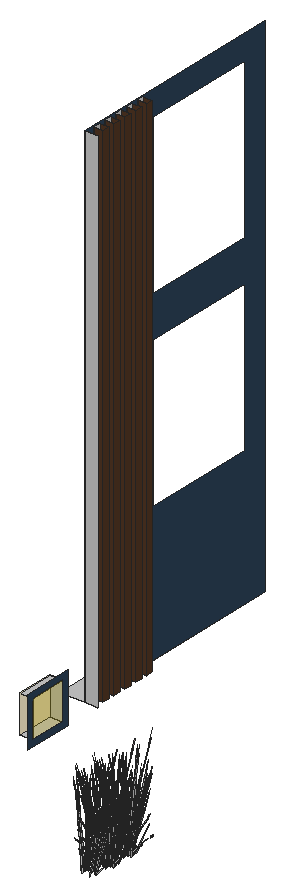
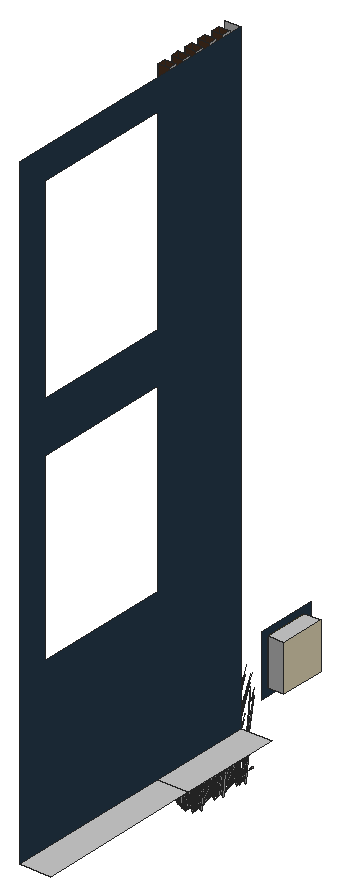
# SketchUp Ruby script. Lengths in inches.
U = 1.inch
M = Sketchup.active_model
def pt(a) = Geom::Point3d.new(a.map { |v| v * U })
def face(e, loops, mat)
  f = e.add_face(loops[0].map { |a| pt(a) })
  loops[1..].each { |l| e.add_face(l.map { |a| pt(a) }).erase! }
  f.material = f.back_material = mat if mat
  f
end
# faces: each face lists its corners as indices into pts; further lists are holes
def faces(e, pts, list, mat = nil) = list.each { |f| face(e, (f[0].is_a?(Array) ? f : [f]).map { |l| l.map { |i| pts[i] } }, mat) }
# xy, xz, yz: faces in a plane at the given z, y or x. An outline is a flat list of corners, or four numbers for a rectangle; further outlines are holes
def ring(l) = l.size == 4 ? [[l[0], l[1]], [l[2], l[1]], [l[2], l[3]], [l[0], l[3]]] : l.each_slice(2).to_a
def flat(e, list, mat, &to3) = list.each { |f| face(e, (f[0].is_a?(Array) ? f : [f]).map { |l| ring(l).map { |u, v| to3.(u, v) } }, mat) }
def xy(e, z, list, mat = nil) = flat(e, list, mat) { |x, y| [x, y, z] }
def xz(e, y, list, mat = nil) = flat(e, list, mat) { |x, z| [x, y, z] }
def yz(e, x, list, mat = nil) = flat(e, list, mat) { |y, z| [x, y, z] }
def lines(e, pts, list) = list.each { |a, b| e.add_line(pt(pts[a]), pt(pts[b])) }
# prism: a flat outline (further loops are holes) pulled along v
def prism(e, loops, v, mat = nil)
  f = face(e, loops, mat); d = Geom::Vector3d.new(v.map { |x| x * U })
  f.pushpull(f.normal.samedirection?(d) ? d.length : -d.length)
end
def box(e, o, s, mat = nil) = prism(e, [[o, [o[0] + s[0], o[1], o[2]], [o[0] + s[0], o[1] + s[1], o[2]], [o[0], o[1] + s[1], o[2]]]], [0, 0, s[2]], mat)
def at(x, y, z, deg = 0) = Geom::Transformation.translation(pt([x, y, z])) * Geom::Transformation.rotation(ORIGIN, Z_AXIS, deg.degrees)
def axes(o, x, y, z) = Geom::Transformation.new([*x, 0, *y, 0, *z, 0, *pt(o).to_a, 1])
def part(name) = M.definitions.add(name)
# library, detail: a bought-in or finely detailed component or shape, given as its bounding box
def library(name, o, s) = part(name).tap { |d| box(d.entities, o, s) }
def detail(e, o, s) = box(e.add_group.entities, o, s)
def put(e, d, t, mat = nil) = e.add_instance(d, t).tap { |i| i.material = mat if mat }
def group(e, t, mat = nil) = e.add_group.tap { |g| g.transformation = t; g.material = mat if mat }.entities
root = M.entities
M.materials.add("Carpet_04_1K").color = [43, 65, 85]
M.materials.add("D01_Frost_White").color = [255, 242, 206]
M.materials.add("Glass_Basic_01").color = [255, 228, 0]
M.materials["Glass_Basic_01"].alpha = 0.25
M.materials.add("LightPink_Translucent").color = [144, 107, 117]
M.materials["LightPink_Translucent"].alpha = 0.75
M.materials.add("Wood_Veneer_15_1K").color = [81, 54, 35]
M.materials.add("[_0053_Ivory_]").color = [200, 200, 200]
c1 = part("blade")
p = [[2.15,0.21,22],[0,0.17,0],[0.09,0.45,0],[2.18,0.31,22],[2.29,0.31,22],[0.38,0.45,0],
  [2.48,0.24,33],[2.49,0.24,33],[2.48,0.22,33]]
faces(c1.entities,p,[[0,1,2,3],[4,5,2,3],[6,3,4,7],[8,0,3,6]])
c2 = part("seeds")
p = [[0.3,-0.1,1.38],[-0.01,-0.03,1.59],[-0.01,-0.03,0.03],[0.14,-0.07,-0.07],[0.29,-0.03,3],[0.15,0.01,3.11]]
faces(c2.entities,p,[[0,1,2,3],[1,0,4,5]],"LightPink_Translucent")
c3 = part("blade with seeds")
put(c3.entities,c1,at(0,0,0))
put(c3.entities,c2,axes([2.4,0.25,30.99],[1.5799,-0.05474,1.17369],[-0.12525,1.92788,0.29478],[-0.07173,-0.02425,1.56792]))
xy(root,84,[[635.1,371.15,647.1,411.95],[648.1,375.42,652.51,378.69],[648.1,381.96,652.51,385.24],[648.1,388.51,652.51,391.78],[648.1,395.05,652.51,398.33],
  [648.1,401.6,652.51,404.87],[635.1,411.95,647.1,479.15]],"[_0053_Ivory_]")
xy(root,87,[[647.1,332.15,653.51,350.15]],"[_0053_Ivory_]")
xy(root,105,[[647.1,332.15,653.51,350.15]],"[_0053_Ivory_]")
xz(root,350.15,[[647.1,87,653.51,105]],"[_0053_Ivory_]")
xz(root,371.15,[[647.1,84,653.51,330]],"[_0053_Ivory_]")
xz(root,375.42,[[648.1,84,652.51,330]],"Wood_Veneer_15_1K")
xz(root,378.69,[[648.1,84,652.51,330]],"Wood_Veneer_15_1K")
xz(root,381.96,[[648.1,84,652.51,330]],"Wood_Veneer_15_1K")
xz(root,385.24,[[648.1,84,652.51,330]],"Wood_Veneer_15_1K")
xz(root,388.51,[[648.1,84,652.51,330]],"Wood_Veneer_15_1K")
xz(root,391.78,[[648.1,84,652.51,330]],"Wood_Veneer_15_1K")
xz(root,395.05,[[648.1,84,652.51,330]],"Wood_Veneer_15_1K")
xz(root,398.33,[[648.1,84,652.51,330]],"Wood_Veneer_15_1K")
xz(root,401.6,[[648.1,84,652.51,330]],"Wood_Veneer_15_1K")
xz(root,404.87,[[648.1,84,652.51,330]],"Wood_Veneer_15_1K")
yz(root,647.1,[[[371.15,84,479.15,330],[411.95,241.75,467.15,318],[411.95,150,467.15,222]]],"Carpet_04_1K")
yz(root,647.1,[[332.15,87,350.15,105]],"D01_Frost_White")
yz(root,648.1,[[375.42,84,378.69,330],[381.96,84,385.24,330],[388.51,84,391.78,330],[395.05,84,398.33,330],[401.6,84,404.87,330]],"[_0053_Ivory_]")
yz(root,652.51,[[375.42,84,378.69,330],[381.96,84,385.24,330],[388.51,84,391.78,330],[395.05,84,398.33,330],[401.6,84,404.87,330]],"Wood_Veneer_15_1K")
yz(root,653.51,[[[329.15,84,353.15,108],[332.15,87,350.15,105]]],"Carpet_04_1K")
yz(root,653.51,[[332.15,87,350.15,105]],"Glass_Basic_01")
put(root,c3,axes([677.18,332.05,38.6875],[0.30559,0.56943,-0.1216],[-0.54237,0.27983,-0.67495],[-0.22856,0.07513,1.02557]),"[_0053_Ivory_]")
put(root,c3,axes([681.79,334.5,38.6875],[0.03252,-0.63953,-0.1216],[0.61574,0.01748,-0.67495],[0.23714,0.04442,1.02557]),"[_0053_Ivory_]")
put(root,c3,axes([681.69,334.25,38.7],[-0.34557,-0.39372,0.35414],[0.39459,-0.37271,-0.4572],[0.20048,0.05671,0.87481]),"[_0053_Ivory_]")
put(root,c3,axes([682.32,334.12,38.37],[0.13029,-0.01064,1.74944],[0.35737,-0.48855,-0.27667],[0.23175,0.06449,0.14031]),"[_0053_Ivory_]")
put(root,c3,axes([677.11,333.64,38.39],[-0.15063,-0.57876,0.48003],[0.59087,-0.10045,0.3958],[-0.17414,0.13612,0.9933]),"[_0053_Ivory_]")
put(root,c3,axes([677,333.53,38.38],[-0.41695,-0.26447,0.0643],[0.24275,-0.37662,0.50621],[-0.13368,0.12176,0.77189]),"[_0053_Ivory_]")
put(root,c3,axes([679.55,339.63,38.37],[-0.0929,-0.08817,1.74944],[-0.61994,0.0559,-0.27667],[-0.09894,-0.21089,0.14031]),"[_0053_Ivory_]")
put(root,c3,axes([677.48,333.45,38.7],[0.52868,-0.08987,0.35414],[0.1396,0.51376,-0.4572],[-0.1515,0.13799,0.87481]),"[_0053_Ivory_]")
put(root,c3,axes([675.4375,333.22,38.36],[0.07751,0.01687,1.77383],[0.23978,0.55562,-0.16761],[-0.15867,0.14583,0.31391]),"[_0053_Ivory_]")
put(root,c3,axes([682.01,334.61,38.38],[-0.03058,0.47819,0.0643],[-0.4618,-0.01311,0.50621],[0.1769,0.05004,0.77189]),"[_0053_Ivory_]")
put(root,c3,axes([682.05,334.46,38.39],[-0.44783,0.41436,0.48003],[-0.38623,-0.44004,0.3958],[0.21011,0.07643,0.9933]),"[_0053_Ivory_]")
put(root,c3,axes([682.33,340.71,38.37],[-0.00586,-0.12516,1.74944],[-0.49517,-0.36172,-0.27667],[0.07656,-0.21927,0.14031]),"[_0053_Ivory_]")
put(root,c3,axes([682.2,340.26,38.36],[-0.06168,0.04803,1.77383],[-0.60432,-0.16205,-0.16761],[-0.02188,-0.20961,0.31391]),"[_0053_Ivory_]")
put(root,c3,axes([676.28,334.91,39.3],[0.53595,0.16786,-0.06488],[-0.16486,0.51664,-0.29416],[-0.08766,0.07844,0.97024]),"[_0053_Ivory_]")
put(root,c3,axes([680.625,334.9375,38.7],[-0.0938,-0.50652,0.35414],[0.53623,-0.13375,-0.4572],[0.14403,0.14515,0.87481]),"[_0053_Ivory_]")
put(root,c3,axes([678.91,339.34,38.36],[-0.01133,0.07538,1.77383],[-0.55883,0.27355,-0.16761],[-0.16445,-0.13983,0.31391]),"[_0053_Ivory_]")
put(root,c3,axes([680.98,332.02,38.13],[-0.52482,-0.32674,1.38283],[0.55416,-0.50872,0.59665],[0.16933,0.30658,1.33663]),"[_0053_Ivory_]")
put(root,c3,axes([677.2,333.4,38.6875],[0.56181,0.34675,-0.1216],[-0.32367,0.50216,-0.67495],[-0.15873,0.17455,1.02557]),"[_0053_Ivory_]")
put(root,c3,axes([678.79,340.68,38.75],[0.67657,-0.16163,0.53763],[0.11742,0.63404,0.4433],[-0.15912,-0.18687,1.11249]),"[_0053_Ivory_]")
put(root,c3,axes([680.57,335.2,38.6875],[0.36191,-0.53827,-0.1216],[0.52412,0.3101,-0.67495],[0.18219,0.15207,1.02557]),"[_0053_Ivory_]")
put(root,c3,axes([680.32,340.8,38.39],[0.59846,0.1644,0.48003],[-0.20464,0.54049,0.3958],[-0.03596,-0.21255,0.9933]),"[_0053_Ivory_]")
put(root,c3,axes([680.49,340.99,38.6875],[-0.59433,0.29278,-0.1216],[-0.29207,-0.51964,-0.67495],[-0.07842,-0.21898,1.02557]),"[_0053_Ivory_]")
put(root,c3,axes([681.72,341.65,38.6875],[-0.6675,-0.03116,-0.1216],[0.01824,-0.58993,-0.67495],[0.04637,-0.2272,1.02557]),"[_0053_Ivory_]")
put(root,c3,axes([680.48,340.76,38.38],[0.44753,-0.21372,0.0643],[0.21905,0.38973,0.50621],[-0.04322,-0.1718,0.77189]),"[_0053_Ivory_]")
put(root,c3,axes([678.1875,334.47,38.7],[0.41095,-0.33109,0.35414],[0.38901,0.37805,-0.4572],[-0.05919,0.19208,0.87481]),"[_0053_Ivory_]")
put(root,c3,axes([680.1,335.65,38.36],[0.0018,-0.07613,1.77383],[0.52048,-0.3359,-0.16761],[0.18079,0.11989,0.31391]),"[_0053_Ivory_]")
put(root,c3,axes([677.82,334.77,38.38],[-0.49911,-0.0293,0.0643],[0.01368,-0.44245,0.50621],[-0.05223,0.16948,0.77189]),"[_0053_Ivory_]")
put(root,c3,axes([677.98,334.81,38.39],[-0.43249,-0.42907,0.48003],[0.45929,-0.37004,0.3958],[-0.07978,0.2013,0.9933]),"[_0053_Ivory_]")
put(root,c3,axes([679.34,335.02,38.7],[0.1831,-0.48359,0.35414],[0.53419,0.14105,-0.4572],[0.04898,0.1947,0.87481]),"[_0053_Ivory_]")
put(root,c3,axes([678.94,340.82,38.38],[0.27604,-0.39948,0.0643],[0.39309,0.23258,0.50621],[-0.12709,-0.12808,0.77189]),"[_0053_Ivory_]")
put(root,c3,axes([680.71,335.4,38.38],[-0.27604,0.39948,0.0643],[-0.39309,-0.23258,0.50621],[0.12709,0.12808,0.77189]),"[_0053_Ivory_]")
put(root,c3,axes([680.06,336.74,39.3],[0.4197,-0.36076,-0.06488],[0.38456,0.39511,-0.29416],[0.02707,0.11196,0.97024]),"[_0053_Ivory_]")
put(root,c3,axes([680.31,341.2,38.7],[-0.1831,0.48359,0.35414],[-0.53419,-0.14105,-0.4572],[-0.04898,-0.1947,0.87481]),"[_0053_Ivory_]")
put(root,c3,axes([680.82,335.29,38.39],[-0.60408,0.14432,0.48003],[-0.10484,-0.56611,0.3958],[0.14207,0.16684,0.9933]),"[_0053_Ivory_]")
put(root,c3,axes([681.68,341.4,38.39],[0.43249,0.42907,0.48003],[-0.45929,0.37004,0.3958],[0.07978,-0.2013,0.9933]),"[_0053_Ivory_]")
put(root,c3,axes([679.07,340.78,39.08],[-0.40534,0.60286,-0.13619],[-0.58702,-0.34732,-0.75594],[-0.20405,-0.17032,1.14864]),"[_0053_Ivory_]")
put(root,c3,axes([681.84,341.44,38.38],[0.49911,0.0293,0.0643],[-0.01368,0.44245,0.50621],[0.05223,-0.16948,0.77189]),"[_0053_Ivory_]")
put(root,c3,axes([681.46,341.74,38.7],[-0.41095,0.33109,0.35414],[-0.38901,-0.37805,-0.4572],[0.05919,-0.19208,0.87481]),"[_0053_Ivory_]")
put(root,c3,axes([679.18,335.46,38.38],[-0.44753,0.21372,0.0643],[-0.21905,-0.38973,0.50621],[0.04322,0.1718,0.77189]),"[_0053_Ivory_]")
put(root,c3,axes([676.56,334.85,38.37],[-0.0151,0.12444,1.74944],[0.42844,0.43292,-0.27667],[-0.11216,0.20472,0.14031]),"[_0053_Ivory_]")
put(root,c3,axes([677.93,334.56,39.05],[0.6675,0.03116,-0.13498],[-0.01824,0.58993,-0.74919],[-0.04637,0.2272,1.13838]),"[_0053_Ivory_]")
put(root,c3,axes([679.16,335.22,38.6875],[0.59433,-0.29278,-0.1216],[0.29207,0.51964,-0.67495],[0.07842,0.21898,1.02557]),"[_0053_Ivory_]")
put(root,c3,axes([679.33,335.42,38.72],[-0.59846,-0.1644,0.53283],[0.20464,-0.54049,0.43934],[0.03596,0.21255,1.10256]),"[_0053_Ivory_]")
put(root,c3,axes([677.51,340.6,38.37],[-0.13068,-0.00444,1.74944],[-0.41604,0.44388,-0.27667],[-0.22198,-0.0907,0.14031]),"[_0053_Ivory_]")
put(root,c3,axes([682.45,342.8125,38.6875],[-0.56181,-0.34675,-0.1216],[0.32367,-0.50216,-0.67495],[0.15873,-0.17455,1.02557]),"[_0053_Ivory_]")
put(root,c3,axes([679.03,341.28,38.7],[0.0938,0.50652,0.35414],[-0.53623,0.13375,-0.4572],[-0.14403,-0.14515,0.87481]),"[_0053_Ivory_]")
put(root,c3,axes([677.42,341.61,38.75],[0.50157,-0.46409,0.53763],[0.43258,0.49285,0.4433],[-0.23532,-0.08561,1.11249]),"[_0053_Ivory_]")
put(root,c3,axes([683.83,342.66,38.36],[-0.07933,-0.00478,1.77383],[-0.32942,-0.51175,-0.16761],[0.13229,-0.16826,0.31391]),"[_0053_Ivory_]")
put(root,c3,axes([676.51,336.12,38.36],[0.0689,-0.03797,1.77383],[0.5695,0.25254,-0.16761],[-0.01338,0.21027,0.31391]),"[_0053_Ivory_]")
put(root,c3,axes([677.65,341.6,38.38],[0.03058,-0.47819,0.0643],[0.4618,0.01311,0.50621],[-0.1769,-0.05004,0.77189]),"[_0053_Ivory_]")
put(root,c3,axes([682.18,342.77,38.7],[-0.52868,0.08987,0.35414],[-0.1396,-0.51376,-0.4572],[0.1515,-0.13799,0.87481]),"[_0053_Ivory_]")
put(root,c3,axes([679.02,336.39,38.37],[0.07699,0.10127,1.74944],[0.6213,0.03978,-0.27667],[0.06248,0.22333,0.14031]),"[_0053_Ivory_]")
put(root,c3,axes([682.66,342.68,38.38],[0.41695,0.26447,0.0643],[-0.24275,0.37662,0.50621],[0.13368,-0.12176,0.77189]),"[_0053_Ivory_]")
put(root,c3,axes([682.54,342.57,38.39],[0.15063,0.57876,0.48003],[-0.59087,0.10045,0.3958],[0.17414,-0.13612,0.9933]),"[_0053_Ivory_]")
put(root,c3,axes([684.13,343.27,38.37],[0.08428,-0.09579,1.74944],[-0.10787,-0.58756,-0.27667],[0.21147,-0.1114,0.14031]),"[_0053_Ivory_]")
put(root,c3,axes([677.01,340.98,38.36],[0.04503,0.06276,1.77383],[-0.21706,0.56413,-0.16761],[-0.21983,0.00408,0.31391]),"[_0053_Ivory_]")
put(root,c3,axes([677.96,341.96,38.7],[0.34557,0.39372,0.35414],[-0.39459,0.37271,-0.4572],[-0.20048,-0.05671,0.87481]),"[_0053_Ivory_]")
put(root,c3,axes([677.87,341.71,38.6875],[-0.03252,0.63953,-0.1216],[-0.61574,-0.01748,-0.67495],[-0.23714,-0.04442,1.02557]),"[_0053_Ivory_]")
put(root,c3,axes([682.47,344.17,38.6875],[-0.30559,-0.56943,-0.1216],[0.54237,-0.27983,-0.67495],[0.22856,-0.07513,1.02557]),"[_0053_Ivory_]")
put(root,c3,axes([682.26,343.99,38.7],[-0.50475,-0.17543,0.35414],[0.14722,-0.5118,-0.4572],[0.20322,-0.04693,0.87481]),"[_0053_Ivory_]")
put(root,c3,axes([676.98,343.06,38.39],[0.17159,-0.57338,0.48003],[0.56413,0.19607,0.3958],[-0.22185,0.03446,0.9933]),"[_0053_Ivory_]")
put(root,c3,axes([676.93,342.91,38.38],[-0.22307,-0.42878,0.0643],[0.40677,-0.20987,0.50621],[-0.17931,0.04141,0.77189]),"[_0053_Ivory_]")
put(root,c3,axes([682.72,344.15,38.38],[0.22307,0.42878,0.0643],[-0.40677,0.20987,0.50621],[0.17931,-0.04141,0.77189]),"[_0053_Ivory_]")
put(root,c3,axes([682.68,344,38.39],[-0.17159,0.57338,0.48003],[-0.56413,-0.19607,0.3958],[0.22185,-0.03446,0.9933]),"[_0053_Ivory_]")
put(root,c3,axes([677.39,343.07,38.7],[0.50475,0.17543,0.35414],[-0.14722,0.5118,-0.4572],[-0.20322,0.04693,0.87481]),"[_0053_Ivory_]")
put(root,c3,axes([683.6875,345.86,38.36],[-0.05492,-0.05505,1.77383],[0.12013,-0.59013,-0.16761],[0.21632,-0.0377,0.31391]),"[_0053_Ivory_]")
put(root,c3,axes([676.54,343.46,38.37],[-0.09918,0.08165,1.74944],[0.00844,0.59653,-0.27667],[-0.22734,0.07758,0.14031]),"[_0053_Ivory_]")
put(root,c3,axes([677.18,342.89,38.6875],[0.30559,0.56943,-0.1216],[-0.54237,0.27983,-0.67495],[-0.22856,0.07513,1.02557]),"[_0053_Ivory_]")
put(root,c3,axes([681.79,345.35,38.6875],[0.03252,-0.63953,-0.1216],[0.61574,0.01748,-0.67495],[0.23714,0.04442,1.02557]),"[_0053_Ivory_]")
put(root,c3,axes([681.69,345.1,38.7],[-0.34557,-0.39372,0.35414],[0.39459,-0.37271,-0.4572],[0.20048,0.05671,0.87481]),"[_0053_Ivory_]")
put(root,c3,axes([682.32,344.96,38.37],[0.13029,-0.01064,1.74944],[0.35737,-0.48855,-0.27667],[0.23175,0.06449,0.14031]),"[_0053_Ivory_]")
put(root,c3,axes([677.11,344.49,38.39],[-0.15063,-0.57876,0.48003],[0.59087,-0.10045,0.3958],[-0.17414,0.13612,0.9933]),"[_0053_Ivory_]")
put(root,c3,axes([677,344.375,38.38],[-0.41695,-0.26447,0.0643],[0.24275,-0.37662,0.50621],[-0.13368,0.12176,0.77189]),"[_0053_Ivory_]")
put(root,c3,axes([679.55,350.3,38.37],[-0.0929,-0.08817,1.74944],[-0.61994,0.0559,-0.27667],[-0.09894,-0.21089,0.14031]),"[_0053_Ivory_]")
put(root,c3,axes([677.48,344.29,38.7],[0.52868,-0.08987,0.35414],[0.1396,0.51376,-0.4572],[-0.1515,0.13799,0.87481]),"[_0053_Ivory_]")
put(root,c3,axes([675.4375,344.07,38.36],[0.07751,0.01687,1.77383],[0.23978,0.55562,-0.16761],[-0.15867,0.14583,0.31391]),"[_0053_Ivory_]")
put(root,c3,axes([682.01,345.45,38.38],[-0.03058,0.47819,0.0643],[-0.4618,-0.01311,0.50621],[0.1769,0.05004,0.77189]),"[_0053_Ivory_]")
put(root,c3,axes([682.33,351.38,38.37],[-0.00586,-0.12516,1.74944],[-0.49517,-0.36172,-0.27667],[0.07656,-0.21927,0.14031]),"[_0053_Ivory_]")
put(root,c3,axes([682.2,350.93,38.36],[-0.06168,0.04803,1.77383],[-0.60432,-0.16205,-0.16761],[-0.02188,-0.20961,0.31391]),"[_0053_Ivory_]")
put(root,c3,axes([682.05,345.3,38.39],[-0.44783,0.41436,0.48003],[-0.38623,-0.44004,0.3958],[0.21011,0.07643,0.9933]),"[_0053_Ivory_]")
put(root,c3,axes([676.28,345.75,39.3],[0.53595,0.16786,-0.06488],[-0.16486,0.51664,-0.29416],[-0.08766,0.07844,0.97024]),"[_0053_Ivory_]")
put(root,c3,axes([678.91,350.01,38.36],[-0.01133,0.07538,1.77383],[-0.55883,0.27355,-0.16761],[-0.16445,-0.13983,0.31391]),"[_0053_Ivory_]")
put(root,c3,axes([680.625,345.78,38.7],[-0.0938,-0.50652,0.35414],[0.53623,-0.13375,-0.4572],[0.14403,0.14515,0.87481]),"[_0053_Ivory_]")
put(root,c3,axes([680.98,342.87,38.13],[-0.52482,-0.32674,1.38283],[0.55416,-0.50872,0.59665],[0.16933,0.30658,1.33663]),"[_0053_Ivory_]")
put(root,c3,axes([678.79,351.35,38.75],[0.67657,-0.16163,0.53763],[0.11742,0.63404,0.4433],[-0.15912,-0.18687,1.11249]),"[_0053_Ivory_]")
put(root,c3,axes([680.32,351.47,38.39],[0.59846,0.1644,0.48003],[-0.20464,0.54049,0.3958],[-0.03596,-0.21255,0.9933]),"[_0053_Ivory_]")
put(root,c3,axes([680.49,351.66,38.6875],[-0.59433,0.29278,-0.1216],[-0.29207,-0.51964,-0.67495],[-0.07842,-0.21898,1.02557]),"[_0053_Ivory_]")
put(root,c3,axes([677.2,344.25,38.6875],[0.56181,0.34675,-0.1216],[-0.32367,0.50216,-0.67495],[-0.15873,0.17455,1.02557]),"[_0053_Ivory_]")
put(root,c3,axes([681.72,352.32,38.6875],[-0.6675,-0.03116,-0.1216],[0.01824,-0.58993,-0.67495],[0.04637,-0.2272,1.02557]),"[_0053_Ivory_]")
put(root,c3,axes([680.57,346.04,38.6875],[0.36191,-0.53827,-0.1216],[0.52412,0.3101,-0.67495],[0.18219,0.15207,1.02557]),"[_0053_Ivory_]")
put(root,c3,axes([680.48,351.43,38.38],[0.44753,-0.21372,0.0643],[0.21905,0.38973,0.50621],[-0.04322,-0.1718,0.77189]),"[_0053_Ivory_]")
put(root,c3,axes([678.1875,345.32,38.7],[0.41095,-0.33109,0.35414],[0.38901,0.37805,-0.4572],[-0.05919,0.19208,0.87481]),"[_0053_Ivory_]")
put(root,c3,axes([680.1,346.49,38.36],[0.0018,-0.07613,1.77383],[0.52048,-0.3359,-0.16761],[0.18079,0.11989,0.31391]),"[_0053_Ivory_]")
put(root,c3,axes([677.82,345.62,38.38],[-0.49911,-0.0293,0.0643],[0.01368,-0.44245,0.50621],[-0.05223,0.16948,0.77189]),"[_0053_Ivory_]")
put(root,c3,axes([677.98,345.66,38.39],[-0.43249,-0.42907,0.48003],[0.45929,-0.37004,0.3958],[-0.07978,0.2013,0.9933]),"[_0053_Ivory_]")
put(root,c3,axes([678.94,351.49,38.38],[0.27604,-0.39948,0.0643],[0.39309,0.23258,0.50621],[-0.12709,-0.12808,0.77189]),"[_0053_Ivory_]")
put(root,c3,axes([679.34,345.86,38.7],[0.1831,-0.48359,0.35414],[0.53419,0.14105,-0.4572],[0.04898,0.1947,0.87481]),"[_0053_Ivory_]")
put(root,c3,axes([680.31,351.86,38.7],[-0.1831,0.48359,0.35414],[-0.53419,-0.14105,-0.4572],[-0.04898,-0.1947,0.87481]),"[_0053_Ivory_]")
put(root,c3,axes([680.71,346.24,38.38],[-0.27604,0.39948,0.0643],[-0.39309,-0.23258,0.50621],[0.12709,0.12808,0.77189]),"[_0053_Ivory_]")
put(root,c3,axes([681.68,352.07,38.39],[0.43249,0.42907,0.48003],[-0.45929,0.37004,0.3958],[0.07978,-0.2013,0.9933]),"[_0053_Ivory_]")
put(root,c3,axes([679.07,351.44,39.08],[-0.40534,0.60286,-0.13619],[-0.58702,-0.34732,-0.75594],[-0.20405,-0.17032,1.14864]),"[_0053_Ivory_]")
put(root,c3,axes([681.84,352.11,38.38],[0.49911,0.0293,0.0643],[-0.01368,0.44245,0.50621],[0.05223,-0.16948,0.77189]),"[_0053_Ivory_]")
put(root,c3,axes([680.06,347.59,39.3],[0.4197,-0.36076,-0.06488],[0.38456,0.39511,-0.29416],[0.02707,0.11196,0.97024]),"[_0053_Ivory_]")
put(root,c3,axes([680.82,346.13,38.39],[-0.60408,0.14432,0.48003],[-0.10484,-0.56611,0.3958],[0.14207,0.16684,0.9933]),"[_0053_Ivory_]")
put(root,c3,axes([681.46,352.41,38.7],[-0.41095,0.33109,0.35414],[-0.38901,-0.37805,-0.4572],[0.05919,-0.19208,0.87481]),"[_0053_Ivory_]")
put(root,c3,axes([679.18,346.3,38.38],[-0.44753,0.21372,0.0643],[-0.21905,-0.38973,0.50621],[0.04322,0.1718,0.77189]),"[_0053_Ivory_]")
put(root,c3,axes([676.56,345.6875,38.37],[-0.0151,0.12444,1.74944],[0.42844,0.43292,-0.27667],[-0.11216,0.20472,0.14031]),"[_0053_Ivory_]")
put(root,c3,axes([677.93,345.41,39.05],[0.6675,0.03116,-0.13498],[-0.01824,0.58993,-0.74919],[-0.04637,0.2272,1.13838]),"[_0053_Ivory_]")
put(root,c3,axes([677.51,351.27,38.37],[-0.13068,-0.00444,1.74944],[-0.41604,0.44388,-0.27667],[-0.22198,-0.0907,0.14031]),"[_0053_Ivory_]")
put(root,c3,axes([682.45,353.48,38.6875],[-0.56181,-0.34675,-0.1216],[0.32367,-0.50216,-0.67495],[0.15873,-0.17455,1.02557]),"[_0053_Ivory_]")
put(root,c3,axes([679.16,346.07,38.6875],[0.59433,-0.29278,-0.1216],[0.29207,0.51964,-0.67495],[0.07842,0.21898,1.02557]),"[_0053_Ivory_]")
put(root,c3,axes([679.33,346.26,38.72],[-0.59846,-0.1644,0.53283],[0.20464,-0.54049,0.43934],[0.03596,0.21255,1.10256]),"[_0053_Ivory_]")
put(root,c3,axes([679.03,351.94,38.7],[0.0938,0.50652,0.35414],[-0.53623,0.13375,-0.4572],[-0.14403,-0.14515,0.87481]),"[_0053_Ivory_]")
put(root,c3,axes([677.42,352.27,38.75],[0.50157,-0.46409,0.53763],[0.43258,0.49285,0.4433],[-0.23532,-0.08561,1.11249]),"[_0053_Ivory_]")
put(root,c3,axes([683.83,353.33,38.36],[-0.07933,-0.00478,1.77383],[-0.32942,-0.51175,-0.16761],[0.13229,-0.16826,0.31391]),"[_0053_Ivory_]")
put(root,c3,axes([677.65,352.27,38.38],[0.03058,-0.47819,0.0643],[0.4618,0.01311,0.50621],[-0.1769,-0.05004,0.77189]),"[_0053_Ivory_]")
put(root,c3,axes([676.51,346.97,38.36],[0.0689,-0.03797,1.77383],[0.5695,0.25254,-0.16761],[-0.01338,0.21027,0.31391]),"[_0053_Ivory_]")
put(root,c3,axes([682.18,353.43,38.7],[-0.52868,0.08987,0.35414],[-0.1396,-0.51376,-0.4572],[0.1515,-0.13799,0.87481]),"[_0053_Ivory_]")
put(root,c3,axes([679.02,347.23,38.37],[0.07699,0.10127,1.74944],[0.6213,0.03978,-0.27667],[0.06248,0.22333,0.14031]),"[_0053_Ivory_]")
put(root,c3,axes([682.66,353.35,38.38],[0.41695,0.26447,0.0643],[-0.24275,0.37662,0.50621],[0.13368,-0.12176,0.77189]),"[_0053_Ivory_]")
put(root,c3,axes([682.54,353.24,38.39],[0.15063,0.57876,0.48003],[-0.59087,0.10045,0.3958],[0.17414,-0.13612,0.9933]),"[_0053_Ivory_]")
put(root,c3,axes([684.13,353.94,38.37],[0.08428,-0.09579,1.74944],[-0.10787,-0.58756,-0.27667],[0.21147,-0.1114,0.14031]),"[_0053_Ivory_]")
put(root,c3,axes([677.01,351.65,38.36],[0.04503,0.06276,1.77383],[-0.21706,0.56413,-0.16761],[-0.21983,0.00408,0.31391]),"[_0053_Ivory_]")
put(root,c3,axes([677.96,352.63,38.7],[0.34557,0.39372,0.35414],[-0.39459,0.37271,-0.4572],[-0.20048,-0.05671,0.87481]),"[_0053_Ivory_]")
put(root,c3,axes([677.87,352.38,38.6875],[-0.03252,0.63953,-0.1216],[-0.61574,-0.01748,-0.67495],[-0.23714,-0.04442,1.02557]),"[_0053_Ivory_]")
put(root,c3,axes([682.47,354.83,38.6875],[-0.30559,-0.56943,-0.1216],[0.54237,-0.27983,-0.67495],[0.22856,-0.07513,1.02557]),"[_0053_Ivory_]")
put(root,c3,axes([682.26,354.66,38.7],[-0.50475,-0.17543,0.35414],[0.14722,-0.5118,-0.4572],[0.20322,-0.04693,0.87481]),"[_0053_Ivory_]")
put(root,c3,axes([676.98,353.73,38.39],[0.17159,-0.57338,0.48003],[0.56413,0.19607,0.3958],[-0.22185,0.03446,0.9933]),"[_0053_Ivory_]")
put(root,c3,axes([676.93,353.57,38.38],[-0.22307,-0.42878,0.0643],[0.40677,-0.20987,0.50621],[-0.17931,0.04141,0.77189]),"[_0053_Ivory_]")
put(root,c3,axes([682.72,354.82,38.38],[0.22307,0.42878,0.0643],[-0.40677,0.20987,0.50621],[0.17931,-0.04141,0.77189]),"[_0053_Ivory_]")
put(root,c3,axes([682.68,354.67,38.39],[-0.17159,0.57338,0.48003],[-0.56413,-0.19607,0.3958],[0.22185,-0.03446,0.9933]),"[_0053_Ivory_]")
put(root,c3,axes([677.39,353.73,38.7],[0.50475,0.17543,0.35414],[-0.14722,0.5118,-0.4572],[-0.20322,0.04693,0.87481]),"[_0053_Ivory_]")
put(root,c3,axes([683.6875,356.52,38.36],[-0.05492,-0.05505,1.77383],[0.12013,-0.59013,-0.16761],[0.21632,-0.0377,0.31391]),"[_0053_Ivory_]")
put(root,c3,axes([676.54,354.13,38.37],[-0.09918,0.08165,1.74944],[0.00844,0.59653,-0.27667],[-0.22734,0.07758,0.14031]),"[_0053_Ivory_]")
put(root,c3,axes([677.18,353.5625,38.6875],[0.30559,0.56943,-0.1216],[-0.54237,0.27983,-0.67495],[-0.22856,0.07513,1.02557]),"[_0053_Ivory_]")
put(root,c3,axes([681.79,356.02,38.6875],[0.03252,-0.63953,-0.1216],[0.61574,0.01748,-0.67495],[0.23714,0.04442,1.02557]),"[_0053_Ivory_]")
put(root,c3,axes([681.69,355.76,38.7],[-0.34557,-0.39372,0.35414],[0.39459,-0.37271,-0.4572],[0.20048,0.05671,0.87481]),"[_0053_Ivory_]")
put(root,c3,axes([682.32,355.63,38.37],[0.13029,-0.01064,1.74944],[0.35737,-0.48855,-0.27667],[0.23175,0.06449,0.14031]),"[_0053_Ivory_]")
put(root,c3,axes([677.11,355.15,38.39],[-0.15063,-0.57876,0.48003],[0.59087,-0.10045,0.3958],[-0.17414,0.13612,0.9933]),"[_0053_Ivory_]")
put(root,c3,axes([677,355.04,38.38],[-0.41695,-0.26447,0.0643],[0.24275,-0.37662,0.50621],[-0.13368,0.12176,0.77189]),"[_0053_Ivory_]")
put(root,c3,axes([677.48,354.96,38.7],[0.52868,-0.08987,0.35414],[0.1396,0.51376,-0.4572],[-0.1515,0.13799,0.87481]),"[_0053_Ivory_]")
put(root,c3,axes([675.4375,354.73,38.36],[0.07751,0.01687,1.77383],[0.23978,0.55562,-0.16761],[-0.15867,0.14583,0.31391]),"[_0053_Ivory_]")
put(root,c3,axes([682.01,356.12,38.38],[-0.03058,0.47819,0.0643],[-0.4618,-0.01311,0.50621],[0.1769,0.05004,0.77189]),"[_0053_Ivory_]")
put(root,c3,axes([682.05,355.97,38.39],[-0.44783,0.41436,0.48003],[-0.38623,-0.44004,0.3958],[0.21011,0.07643,0.9933]),"[_0053_Ivory_]")
put(root,c3,axes([676.28,356.42,39.3],[0.53595,0.16786,-0.06488],[-0.16486,0.51664,-0.29416],[-0.08766,0.07844,0.97024]),"[_0053_Ivory_]")
put(root,c3,axes([680.625,356.45,38.7],[-0.0938,-0.50652,0.35414],[0.53623,-0.13375,-0.4572],[0.14403,0.14515,0.87481]),"[_0053_Ivory_]")
put(root,c3,axes([680.98,353.54,38.13],[-0.52482,-0.32674,1.38283],[0.55416,-0.50872,0.59665],[0.16933,0.30658,1.33663]),"[_0053_Ivory_]")
put(root,c3,axes([677.2,354.91,38.6875],[0.56181,0.34675,-0.1216],[-0.32367,0.50216,-0.67495],[-0.15873,0.17455,1.02557]),"[_0053_Ivory_]")
put(root,c3,axes([680.57,356.71,38.6875],[0.36191,-0.53827,-0.1216],[0.52412,0.3101,-0.67495],[0.18219,0.15207,1.02557]),"[_0053_Ivory_]")
put(root,c3,axes([678.1875,355.98,38.7],[0.41095,-0.33109,0.35414],[0.38901,0.37805,-0.4572],[-0.05919,0.19208,0.87481]),"[_0053_Ivory_]")
put(root,c3,axes([680.1,357.16,38.36],[0.0018,-0.07613,1.77383],[0.52048,-0.3359,-0.16761],[0.18079,0.11989,0.31391]),"[_0053_Ivory_]")
put(root,c3,axes([677.82,356.28,38.38],[-0.49911,-0.0293,0.0643],[0.01368,-0.44245,0.50621],[-0.05223,0.16948,0.77189]),"[_0053_Ivory_]")
put(root,c3,axes([677.98,356.33,38.39],[-0.43249,-0.42907,0.48003],[0.45929,-0.37004,0.3958],[-0.07978,0.2013,0.9933]),"[_0053_Ivory_]")
put(root,c3,axes([679.34,356.53,38.7],[0.1831,-0.48359,0.35414],[0.53419,0.14105,-0.4572],[0.04898,0.1947,0.87481]),"[_0053_Ivory_]")
put(root,c3,axes([680.71,356.91,38.38],[-0.27604,0.39948,0.0643],[-0.39309,-0.23258,0.50621],[0.12709,0.12808,0.77189]),"[_0053_Ivory_]")
put(root,c3,axes([680.06,358.25,39.3],[0.4197,-0.36076,-0.06488],[0.38456,0.39511,-0.29416],[0.02707,0.11196,0.97024]),"[_0053_Ivory_]")
put(root,c3,axes([680.82,356.8,38.39],[-0.60408,0.14432,0.48003],[-0.10484,-0.56611,0.3958],[0.14207,0.16684,0.9933]),"[_0053_Ivory_]")
put(root,c3,axes([679.18,356.97,38.38],[-0.44753,0.21372,0.0643],[-0.21905,-0.38973,0.50621],[0.04322,0.1718,0.77189]),"[_0053_Ivory_]")
put(root,c3,axes([676.56,356.36,38.37],[-0.0151,0.12444,1.74944],[0.42844,0.43292,-0.27667],[-0.11216,0.20472,0.14031]),"[_0053_Ivory_]")
put(root,c3,axes([677.93,356.08,39.05],[0.6675,0.03116,-0.13498],[-0.01824,0.58993,-0.74919],[-0.04637,0.2272,1.13838]),"[_0053_Ivory_]")
put(root,c3,axes([679.16,356.73,38.6875],[0.59433,-0.29278,-0.1216],[0.29207,0.51964,-0.67495],[0.07842,0.21898,1.02557]),"[_0053_Ivory_]")
put(root,c3,axes([679.33,356.93,38.72],[-0.59846,-0.1644,0.53283],[0.20464,-0.54049,0.43934],[0.03596,0.21255,1.10256]),"[_0053_Ivory_]")
put(root,c3,axes([676.51,357.63,38.36],[0.0689,-0.03797,1.77383],[0.5695,0.25254,-0.16761],[-0.01338,0.21027,0.31391]),"[_0053_Ivory_]")
put(root,c3,axes([679.02,357.9,38.37],[0.07699,0.10127,1.74944],[0.6213,0.03978,-0.27667],[0.06248,0.22333,0.14031]),"[_0053_Ivory_]")
